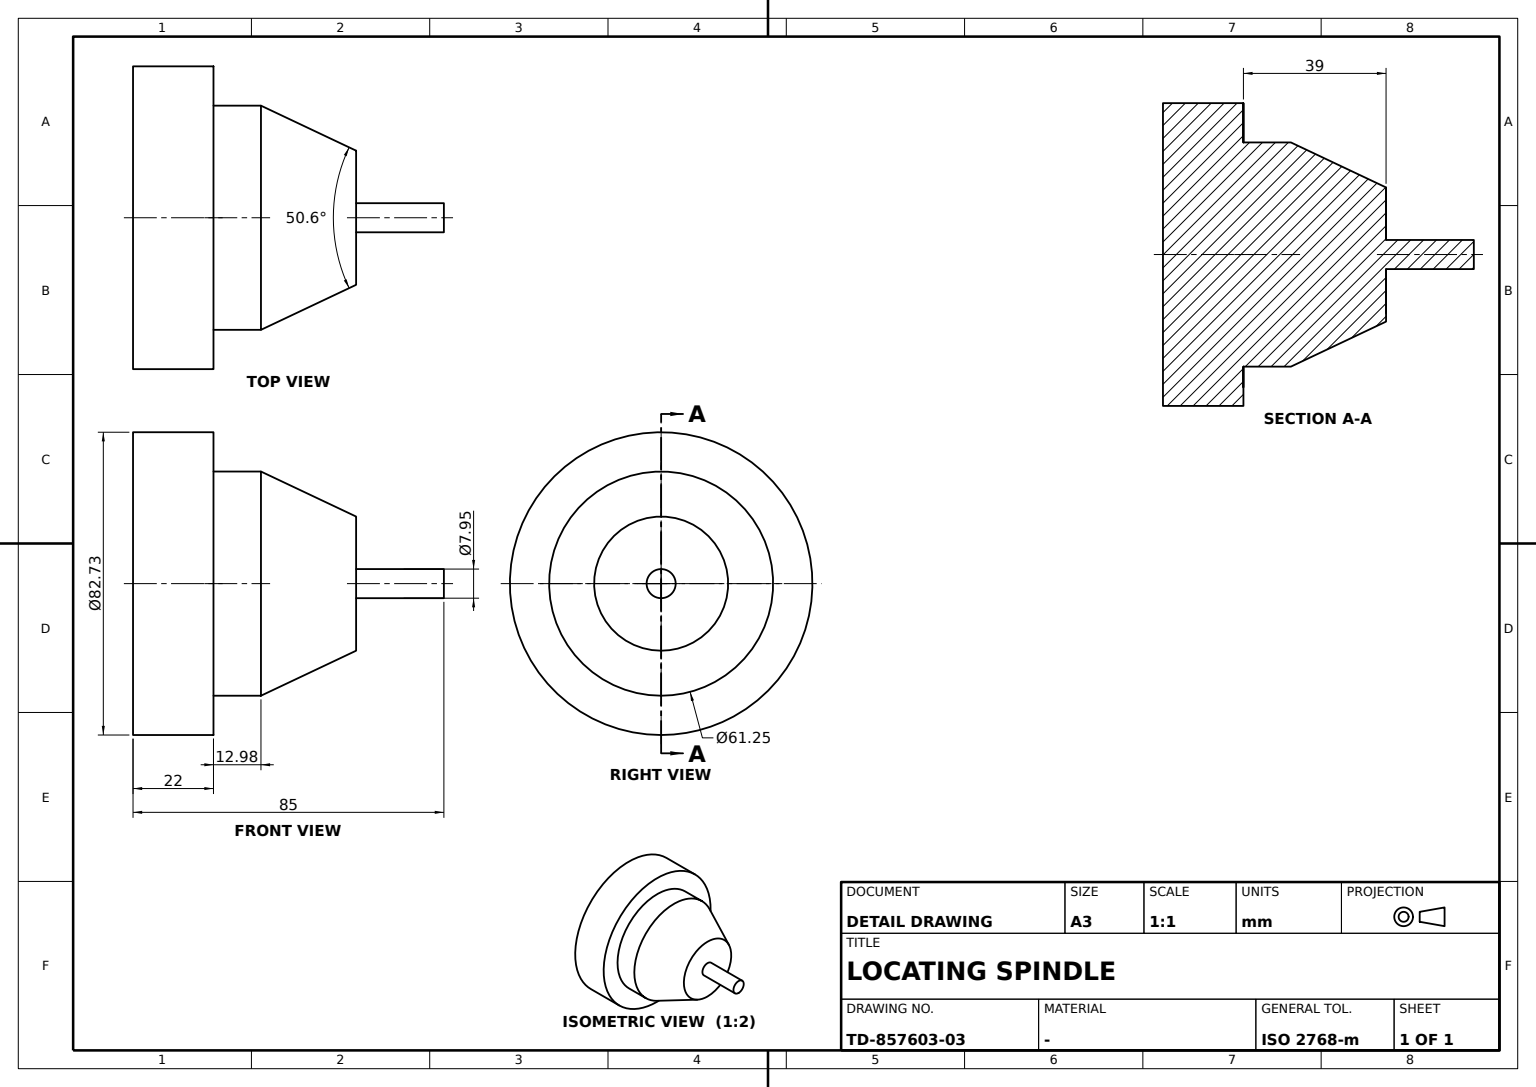
ISO-10303-21;
HEADER;
FILE_DESCRIPTION((''),'2;1');
FILE_NAME('','',(''),(''),'','','');
FILE_SCHEMA(('AUTOMOTIVE_DESIGN'));
ENDSEC;
DATA;
#1=APPLICATION_CONTEXT('');
#2=PRODUCT_CONTEXT('',#1,'mechanical');
#3=PRODUCT('','','',(#2));
#4=PRODUCT_DEFINITION_FORMATION('','',#3);
#5=PRODUCT_DEFINITION_CONTEXT('',#1,'design');
#6=PRODUCT_DEFINITION('','',#4,#5);
#7=PRODUCT_DEFINITION_SHAPE('','',#6);
#8=(LENGTH_UNIT()NAMED_UNIT(*)SI_UNIT(.MILLI.,.METRE.));
#9=(NAMED_UNIT(*)PLANE_ANGLE_UNIT()SI_UNIT($,.RADIAN.));
#10=(NAMED_UNIT(*)SI_UNIT($,.STERADIAN.)SOLID_ANGLE_UNIT());
#11=UNCERTAINTY_MEASURE_WITH_UNIT(LENGTH_MEASURE(1.E-05),#8,'distance_accuracy_value','');
#12=(GEOMETRIC_REPRESENTATION_CONTEXT(3)GLOBAL_UNCERTAINTY_ASSIGNED_CONTEXT((#11))GLOBAL_UNIT_ASSIGNED_CONTEXT((#8,#9,#10))REPRESENTATION_CONTEXT('',''));
#13=CARTESIAN_POINT('',(36.301686,19.831702,-42.534455));
#14=VERTEX_POINT('',#13);
#15=CARTESIAN_POINT('',(36.301686,19.831702,-20.534455));
#16=VERTEX_POINT('',#15);
#17=CARTESIAN_POINT('',(36.301686,19.831702,-31.534455));
#18=DIRECTION('',(0.,0.,1.));
#19=VECTOR('',#18,1000.);
#20=LINE('',#17,#19);
#21=EDGE_CURVE('',#14,#16,#20,.T.);
#22=ORIENTED_EDGE('',*,*,#21,.F.);
#23=CARTESIAN_POINT('',(-36.301686,-19.831702,-42.534455));
#24=VERTEX_POINT('',#23);
#25=CARTESIAN_POINT('',(0.,0.,-42.534455));
#26=DIRECTION('',(1.,0.,0.));
#27=AXIS2_PLACEMENT_3D('',#25,#18,#26);
#28=CIRCLE('',#27,41.365551);
#29=EDGE_CURVE('',#14,#24,#28,.T.);
#30=ORIENTED_EDGE('',*,*,#29,.T.);
#31=CARTESIAN_POINT('',(-36.301686,-19.831702,-20.534455));
#32=VERTEX_POINT('',#31);
#33=CARTESIAN_POINT('',(-36.301686,-19.831702,-31.534455));
#34=LINE('',#33,#19);
#35=EDGE_CURVE('',#24,#32,#34,.T.);
#36=ORIENTED_EDGE('',*,*,#35,.T.);
#37=CARTESIAN_POINT('',(0.,0.,-20.534455));
#38=AXIS2_PLACEMENT_3D('',#37,#18,#26);
#39=CIRCLE('',#38,41.365551);
#40=EDGE_CURVE('',#16,#32,#39,.T.);
#41=ORIENTED_EDGE('',*,*,#40,.F.);
#42=EDGE_LOOP('',(#22,#30,#36,#41));
#43=FACE_OUTER_BOUND('',#42,.T.);
#44=CARTESIAN_POINT('',(0.,0.,-0.034455));
#45=DIRECTION('',(0.,0.,-1.));
#46=AXIS2_PLACEMENT_3D('',#44,#45,#26);
#47=CYLINDRICAL_SURFACE('',#46,41.365551);
#48=ADVANCED_FACE('',(#43),#47,.T.);
#49=ORIENTED_EDGE('',*,*,#40,.T.);
#50=CARTESIAN_POINT('',(41.365551,0.,-20.534455));
#51=VERTEX_POINT('',#50);
#52=EDGE_CURVE('',#32,#51,#39,.T.);
#53=ORIENTED_EDGE('',*,*,#52,.T.);
#54=EDGE_CURVE('',#51,#16,#39,.T.);
#55=ORIENTED_EDGE('',*,*,#54,.T.);
#56=EDGE_LOOP('',(#49,#53,#55));
#57=FACE_OUTER_BOUND('',#56,.T.);
#58=CARTESIAN_POINT('',(26.87721,14.683087,-20.534455));
#59=VERTEX_POINT('',#58);
#60=CARTESIAN_POINT('',(-26.87721,-14.683087,-20.534455));
#61=VERTEX_POINT('',#60);
#62=CIRCLE('',#38,30.626417);
#63=EDGE_CURVE('',#59,#61,#62,.T.);
#64=ORIENTED_EDGE('',*,*,#63,.F.);
#65=CARTESIAN_POINT('',(30.626417,0.,-20.534455));
#66=VERTEX_POINT('',#65);
#67=EDGE_CURVE('',#66,#59,#62,.T.);
#68=ORIENTED_EDGE('',*,*,#67,.F.);
#69=EDGE_CURVE('',#61,#66,#62,.T.);
#70=ORIENTED_EDGE('',*,*,#69,.F.);
#71=EDGE_LOOP('',(#64,#68,#70));
#72=FACE_BOUND('',#71,.T.);
#73=CARTESIAN_POINT('',(-41.365551,0.,-20.534455));
#74=AXIS2_PLACEMENT_3D('',#73,#18,#26);
#75=PLANE('',#74);
#76=ADVANCED_FACE('',(#57,#72),#75,.T.);
#77=CARTESIAN_POINT('',(3.977455,0.,42.465545));
#78=VERTEX_POINT('',#77);
#79=CARTESIAN_POINT('',(3.490545,1.906894,42.465545));
#80=VERTEX_POINT('',#79);
#81=CARTESIAN_POINT('',(0.,0.,42.465545));
#82=AXIS2_PLACEMENT_3D('',#81,#18,#26);
#83=CIRCLE('',#82,3.977455);
#84=EDGE_CURVE('',#78,#80,#83,.T.);
#85=ORIENTED_EDGE('',*,*,#84,.T.);
#86=CARTESIAN_POINT('',(-3.490545,-1.906894,42.465545));
#87=VERTEX_POINT('',#86);
#88=EDGE_CURVE('',#80,#87,#83,.T.);
#89=ORIENTED_EDGE('',*,*,#88,.T.);
#90=EDGE_CURVE('',#87,#78,#83,.T.);
#91=ORIENTED_EDGE('',*,*,#90,.T.);
#92=EDGE_LOOP('',(#85,#89,#91));
#93=FACE_OUTER_BOUND('',#92,.T.);
#94=CARTESIAN_POINT('',(-3.977455,0.,42.465545));
#95=AXIS2_PLACEMENT_3D('',#94,#18,#26);
#96=PLANE('',#95);
#97=ADVANCED_FACE('',(#93),#96,.T.);
#98=CARTESIAN_POINT('',(3.490545,1.906894,18.465545));
#99=VERTEX_POINT('',#98);
#100=CARTESIAN_POINT('',(3.490545,1.906894,30.465545));
#101=LINE('',#100,#19);
#102=EDGE_CURVE('',#99,#80,#101,.T.);
#103=ORIENTED_EDGE('',*,*,#102,.F.);
#104=CARTESIAN_POINT('',(-3.490545,-1.906894,18.465545));
#105=VERTEX_POINT('',#104);
#106=CARTESIAN_POINT('',(0.,0.,18.465545));
#107=AXIS2_PLACEMENT_3D('',#106,#18,#26);
#108=CIRCLE('',#107,3.977455);
#109=EDGE_CURVE('',#99,#105,#108,.T.);
#110=ORIENTED_EDGE('',*,*,#109,.T.);
#111=CARTESIAN_POINT('',(-3.490545,-1.906894,30.465545));
#112=LINE('',#111,#19);
#113=EDGE_CURVE('',#105,#87,#112,.T.);
#114=ORIENTED_EDGE('',*,*,#113,.T.);
#115=ORIENTED_EDGE('',*,*,#88,.F.);
#116=EDGE_LOOP('',(#103,#110,#114,#115));
#117=FACE_OUTER_BOUND('',#116,.T.);
#118=CYLINDRICAL_SURFACE('',#46,3.977455);
#119=ADVANCED_FACE('',(#117),#118,.T.);
#120=ORIENTED_EDGE('',*,*,#29,.F.);
#121=CARTESIAN_POINT('',(41.365551,0.,-42.534455));
#122=VERTEX_POINT('',#121);
#123=EDGE_CURVE('',#122,#14,#28,.T.);
#124=ORIENTED_EDGE('',*,*,#123,.F.);
#125=EDGE_CURVE('',#24,#122,#28,.T.);
#126=ORIENTED_EDGE('',*,*,#125,.F.);
#127=EDGE_LOOP('',(#120,#124,#126));
#128=FACE_OUTER_BOUND('',#127,.T.);
#129=PLANE('',#27);
#130=ADVANCED_FACE('',(#128),#129,.F.);
#131=CARTESIAN_POINT('',(3.977455,0.,18.465545));
#132=VERTEX_POINT('',#131);
#133=CARTESIAN_POINT('',(3.977455,0.,-0.034455));
#134=VECTOR('',#45,1000.);
#135=LINE('',#133,#134);
#136=EDGE_CURVE('',#78,#132,#135,.T.);
#137=ORIENTED_EDGE('',*,*,#136,.F.);
#138=ORIENTED_EDGE('',*,*,#90,.F.);
#139=ORIENTED_EDGE('',*,*,#113,.F.);
#140=EDGE_CURVE('',#105,#132,#108,.T.);
#141=ORIENTED_EDGE('',*,*,#140,.T.);
#142=EDGE_LOOP('',(#137,#138,#139,#141));
#143=FACE_OUTER_BOUND('',#142,.T.);
#144=ADVANCED_FACE('',(#143),#118,.T.);
#145=CARTESIAN_POINT('',(-26.87721,-14.683087,-7.552146));
#146=VERTEX_POINT('',#145);
#147=CARTESIAN_POINT('',(-16.084051,-8.786757,18.465545));
#148=VERTEX_POINT('',#147);
#149=CARTESIAN_POINT('',(-21.48063,-11.734922,5.456699));
#150=DIRECTION('',(0.375047599,0.204889437,0.904079431));
#151=VECTOR('',#150,1000.);
#152=LINE('',#149,#151);
#153=EDGE_CURVE('',#146,#148,#152,.T.);
#154=ORIENTED_EDGE('',*,*,#153,.F.);
#155=CARTESIAN_POINT('',(30.626417,0.,-7.552146));
#156=VERTEX_POINT('',#155);
#157=CARTESIAN_POINT('',(0.,0.,-7.552146));
#158=AXIS2_PLACEMENT_3D('',#157,#18,#26);
#159=CIRCLE('',#158,30.626417);
#160=EDGE_CURVE('',#146,#156,#159,.T.);
#161=ORIENTED_EDGE('',*,*,#160,.T.);
#162=CARTESIAN_POINT('',(18.327678,0.,18.465545));
#163=VERTEX_POINT('',#162);
#164=DIRECTION('',(0.427364462,0.,-0.904079431));
#165=VECTOR('',#164,1000.);
#166=LINE('',#162,#165);
#167=EDGE_CURVE('',#163,#156,#166,.T.);
#168=ORIENTED_EDGE('',*,*,#167,.F.);
#169=CIRCLE('',#107,18.327678);
#170=EDGE_CURVE('',#148,#163,#169,.T.);
#171=ORIENTED_EDGE('',*,*,#170,.F.);
#172=EDGE_LOOP('',(#154,#161,#168,#171));
#173=FACE_OUTER_BOUND('',#172,.T.);
#174=AXIS2_PLACEMENT_3D('',#106,#45,#26);
#175=CONICAL_SURFACE('',#174,18.327678348,0.441575599);
#176=ADVANCED_FACE('',(#173),#175,.T.);
#177=CARTESIAN_POINT('',(26.87721,14.683087,-7.552146));
#178=VERTEX_POINT('',#177);
#179=CARTESIAN_POINT('',(26.87721,14.683087,-14.043301));
#180=LINE('',#179,#19);
#181=EDGE_CURVE('',#59,#178,#180,.T.);
#182=ORIENTED_EDGE('',*,*,#181,.T.);
#183=EDGE_CURVE('',#156,#178,#159,.T.);
#184=ORIENTED_EDGE('',*,*,#183,.F.);
#185=CARTESIAN_POINT('',(30.626417,0.,-0.034455));
#186=LINE('',#185,#134);
#187=EDGE_CURVE('',#156,#66,#186,.T.);
#188=ORIENTED_EDGE('',*,*,#187,.T.);
#189=ORIENTED_EDGE('',*,*,#67,.T.);
#190=EDGE_LOOP('',(#182,#184,#188,#189));
#191=FACE_OUTER_BOUND('',#190,.T.);
#192=CYLINDRICAL_SURFACE('',#46,30.626417);
#193=ADVANCED_FACE('',(#191),#192,.T.);
#194=ORIENTED_EDGE('',*,*,#21,.T.);
#195=ORIENTED_EDGE('',*,*,#54,.F.);
#196=CARTESIAN_POINT('',(41.365551,0.,-0.034455));
#197=LINE('',#196,#134);
#198=EDGE_CURVE('',#51,#122,#197,.T.);
#199=ORIENTED_EDGE('',*,*,#198,.T.);
#200=ORIENTED_EDGE('',*,*,#123,.T.);
#201=EDGE_LOOP('',(#194,#195,#199,#200));
#202=FACE_OUTER_BOUND('',#201,.T.);
#203=ADVANCED_FACE('',(#202),#47,.T.);
#204=EDGE_CURVE('',#178,#146,#159,.T.);
#205=ORIENTED_EDGE('',*,*,#204,.F.);
#206=ORIENTED_EDGE('',*,*,#181,.F.);
#207=ORIENTED_EDGE('',*,*,#63,.T.);
#208=CARTESIAN_POINT('',(-26.87721,-14.683087,-14.043301));
#209=LINE('',#208,#19);
#210=EDGE_CURVE('',#61,#146,#209,.T.);
#211=ORIENTED_EDGE('',*,*,#210,.T.);
#212=EDGE_LOOP('',(#205,#206,#207,#211));
#213=FACE_OUTER_BOUND('',#212,.T.);
#214=ADVANCED_FACE('',(#213),#192,.T.);
#215=CARTESIAN_POINT('',(16.084051,8.786757,18.465545));
#216=VERTEX_POINT('',#215);
#217=CARTESIAN_POINT('',(21.48063,11.734922,5.456699));
#218=DIRECTION('',(-0.375047599,-0.204889437,0.904079431));
#219=VECTOR('',#218,1000.);
#220=LINE('',#217,#219);
#221=EDGE_CURVE('',#178,#216,#220,.T.);
#222=ORIENTED_EDGE('',*,*,#221,.T.);
#223=EDGE_CURVE('',#163,#216,#169,.T.);
#224=ORIENTED_EDGE('',*,*,#223,.F.);
#225=ORIENTED_EDGE('',*,*,#167,.T.);
#226=ORIENTED_EDGE('',*,*,#183,.T.);
#227=EDGE_LOOP('',(#222,#224,#225,#226));
#228=FACE_OUTER_BOUND('',#227,.T.);
#229=ADVANCED_FACE('',(#228),#175,.T.);
#230=ORIENTED_EDGE('',*,*,#125,.T.);
#231=ORIENTED_EDGE('',*,*,#198,.F.);
#232=ORIENTED_EDGE('',*,*,#52,.F.);
#233=ORIENTED_EDGE('',*,*,#35,.F.);
#234=EDGE_LOOP('',(#230,#231,#232,#233));
#235=FACE_OUTER_BOUND('',#234,.T.);
#236=ADVANCED_FACE('',(#235),#47,.T.);
#237=ORIENTED_EDGE('',*,*,#204,.T.);
#238=ORIENTED_EDGE('',*,*,#153,.T.);
#239=EDGE_CURVE('',#216,#148,#169,.T.);
#240=ORIENTED_EDGE('',*,*,#239,.F.);
#241=ORIENTED_EDGE('',*,*,#221,.F.);
#242=EDGE_LOOP('',(#237,#238,#240,#241));
#243=FACE_OUTER_BOUND('',#242,.T.);
#244=ADVANCED_FACE('',(#243),#175,.T.);
#245=ORIENTED_EDGE('',*,*,#210,.F.);
#246=ORIENTED_EDGE('',*,*,#69,.T.);
#247=ORIENTED_EDGE('',*,*,#187,.F.);
#248=ORIENTED_EDGE('',*,*,#160,.F.);
#249=EDGE_LOOP('',(#245,#246,#247,#248));
#250=FACE_OUTER_BOUND('',#249,.T.);
#251=ADVANCED_FACE('',(#250),#192,.T.);
#252=ORIENTED_EDGE('',*,*,#239,.T.);
#253=ORIENTED_EDGE('',*,*,#170,.T.);
#254=ORIENTED_EDGE('',*,*,#223,.T.);
#255=EDGE_LOOP('',(#252,#253,#254));
#256=FACE_OUTER_BOUND('',#255,.T.);
#257=ORIENTED_EDGE('',*,*,#109,.F.);
#258=EDGE_CURVE('',#132,#99,#108,.T.);
#259=ORIENTED_EDGE('',*,*,#258,.F.);
#260=ORIENTED_EDGE('',*,*,#140,.F.);
#261=EDGE_LOOP('',(#257,#259,#260));
#262=FACE_BOUND('',#261,.T.);
#263=CARTESIAN_POINT('',(-18.327678,0.,18.465545));
#264=AXIS2_PLACEMENT_3D('',#263,#18,#26);
#265=PLANE('',#264);
#266=ADVANCED_FACE('',(#256,#262),#265,.T.);
#267=ORIENTED_EDGE('',*,*,#102,.T.);
#268=ORIENTED_EDGE('',*,*,#84,.F.);
#269=ORIENTED_EDGE('',*,*,#136,.T.);
#270=ORIENTED_EDGE('',*,*,#258,.T.);
#271=EDGE_LOOP('',(#267,#268,#269,#270));
#272=FACE_OUTER_BOUND('',#271,.T.);
#273=ADVANCED_FACE('',(#272),#118,.T.);
#274=CLOSED_SHELL('',(#48,#76,#97,#119,#130,#144,#176,#193,#203,#214,#229,#236,#244,#251,#266,#273));
#275=MANIFOLD_SOLID_BREP('',#274);
#276=ADVANCED_BREP_SHAPE_REPRESENTATION('',(#275),#12);
#277=SHAPE_DEFINITION_REPRESENTATION(#7,#276);
ENDSEC;
END-ISO-10303-21;
